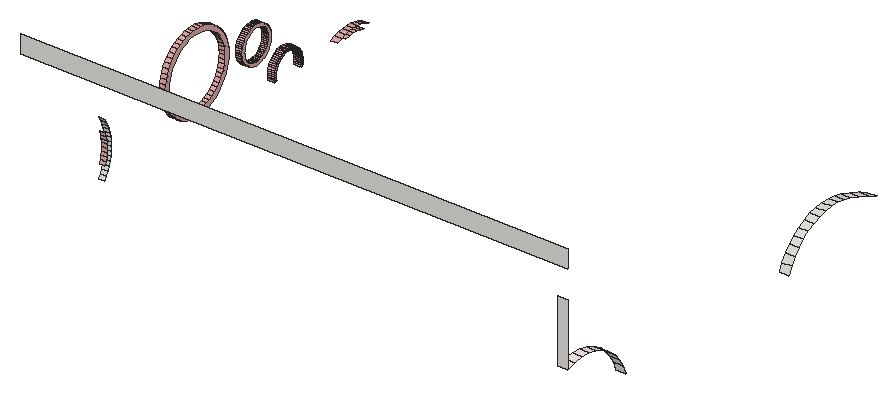
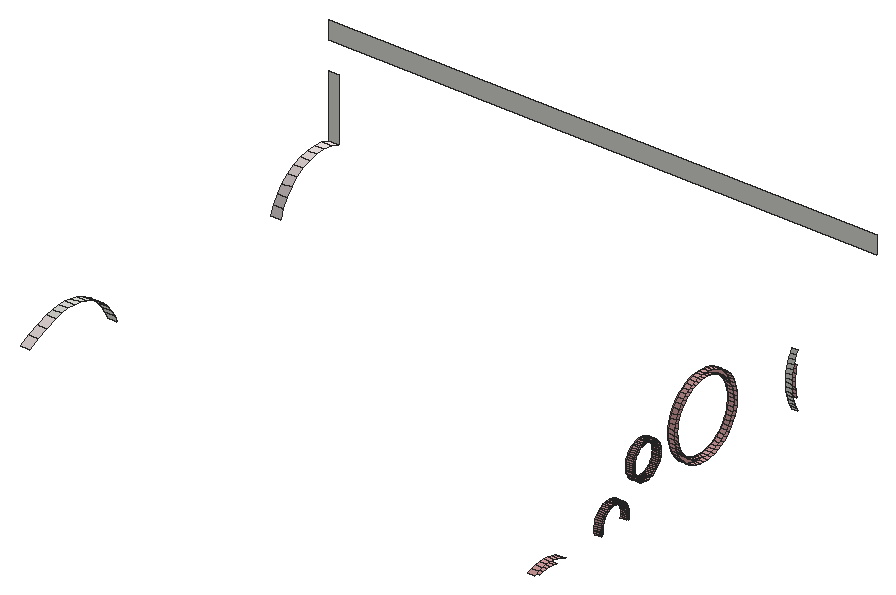
# SketchUp Ruby script. Lengths in inches.
U = 1.inch
M = Sketchup.active_model
def pt(a) = Geom::Point3d.new(a.map { |v| v * U })
def face(e, loops, mat)
  f = e.add_face(loops[0].map { |a| pt(a) })
  loops[1..].each { |l| e.add_face(l.map { |a| pt(a) }).erase! }
  f.material = f.back_material = mat if mat
  f
end
# faces: each face lists its corners as indices into pts; further lists are holes
def faces(e, pts, list, mat = nil) = list.each { |f| face(e, (f[0].is_a?(Array) ? f : [f]).map { |l| l.map { |i| pts[i] } }, mat) }
# xy, xz, yz: faces in a plane at the given z, y or x. An outline is a flat list of corners, or four numbers for a rectangle; further outlines are holes
def ring(l) = l.size == 4 ? [[l[0], l[1]], [l[2], l[1]], [l[2], l[3]], [l[0], l[3]]] : l.each_slice(2).to_a
def flat(e, list, mat, &to3) = list.each { |f| face(e, (f[0].is_a?(Array) ? f : [f]).map { |l| ring(l).map { |u, v| to3.(u, v) } }, mat) }
def xy(e, z, list, mat = nil) = flat(e, list, mat) { |x, y| [x, y, z] }
def xz(e, y, list, mat = nil) = flat(e, list, mat) { |x, z| [x, y, z] }
def yz(e, x, list, mat = nil) = flat(e, list, mat) { |y, z| [x, y, z] }
def lines(e, pts, list) = list.each { |a, b| e.add_line(pt(pts[a]), pt(pts[b])) }
# prism: a flat outline (further loops are holes) pulled along v
def prism(e, loops, v, mat = nil)
  f = face(e, loops, mat); d = Geom::Vector3d.new(v.map { |x| x * U })
  f.pushpull(f.normal.samedirection?(d) ? d.length : -d.length)
end
def box(e, o, s, mat = nil) = prism(e, [[o, [o[0] + s[0], o[1], o[2]], [o[0] + s[0], o[1] + s[1], o[2]], [o[0], o[1] + s[1], o[2]]]], [0, 0, s[2]], mat)
def at(x, y, z, deg = 0) = Geom::Transformation.translation(pt([x, y, z])) * Geom::Transformation.rotation(ORIGIN, Z_AXIS, deg.degrees)
def axes(o, x, y, z) = Geom::Transformation.new([*x, 0, *y, 0, *z, 0, *pt(o).to_a, 1])
def part(name) = M.definitions.add(name)
# library, detail: a bought-in or finely detailed component or shape, given as its bounding box
def library(name, o, s) = part(name).tap { |d| box(d.entities, o, s) }
def detail(e, o, s) = box(e.add_group.entities, o, s)
def put(e, d, t, mat = nil) = e.add_instance(d, t).tap { |i| i.material = mat if mat }
def group(e, t, mat = nil) = e.add_group.tap { |g| g.transformation = t; g.material = mat if mat }.entities
root = M.entities
M.materials.add("Generic").color = [224, 169, 169]
M.materials.add("Generic\#2").color = [246, 234, 234]
xz(root,0,[[180.9375,98.88,184.0625,120],[0,129.25,184.0625,135.25]])
xz(root,88.38,[[10.6875,99.81,12.9375,100.3125]],"Generic")
xz(root,89.3,[[10.6875,99.77,12.9375,100.36]],"Generic")
xz(root,101.73,[[10.6875,86.95,12.9375,87.45]],"Generic")
xz(root,102.58,[[10.6875,86.91,12.9375,87.49]],"Generic")
yz(root,12.625,[[[59.06,89.02,60.53,89.17,61.96,89.47,63.36,89.93,64.7,90.54,65.96,91.29,67.13,92.18,68.2,93.1875,69.15,94.31,69.97,95.53,70.65,96.83,71.18,98.2,71.5625,99.62,71.78,101.07,71.84,102.54,71.74,104,71.48,105.45,71.06,106.86,70.49,108.21,69.77,109.49,68.92,110.6875,67.93,111.78,66.84,112.76,65.64,113.62,64.36,114.33,63.01,114.9,61.6,115.32,60.15,115.58,58.6875,115.68,57.22,115.62,55.77,115.4,54.35,115.02,52.98,114.48,51.68,113.8,50.46,112.98,49.34,112.03,48.33,110.96,47.44,109.79,46.69,108.53,46.08,107.19,45.625,105.8,45.32,104.36,45.18,102.89,45.2,101.43,45.39,99.97,45.73,98.54,46.22,97.16,46.87,95.84,47.66,94.6,48.58,93.45,49.62,92.41,50.76,91.49,52,90.71,53.32,90.0625,54.71,89.57,56.14,89.23,57.6,89.04],[59,90.55,57.7,90.5625,56.41,90.72,55.14,91.03,53.92,91.47,52.75,92.04,51.65,92.73,50.63,93.55,49.71,94.47,48.9,95.48,48.2,96.58,47.63,97.75,47.1875,98.97,46.89,100.24,46.72,101.53,46.71,102.83,46.83,104.13,47.1,105.4,47.5,106.64,48.04,107.82,48.71,108.94,49.49,109.98,50.39,110.93,51.38,111.77,52.46,112.49,53.61,113.1,54.82,113.57,56.08,113.91,57.37,114.11,58.67,114.16,59.96,114.07,61.25,113.84,62.49,113.47,63.69,112.96,64.83,112.33,65.89,111.57,66.86,110.7,67.73,109.74,68.48,108.68,69.12,107.54,69.625,106.34,70,105.1,70.23,103.81,70.32,102.52,70.27,101.22,70.07,99.93,69.73,98.67,69.26,97.46,68.66,96.31,67.93,95.23,67.09,94.23,66.15,93.34,65.11,92.55,63.99,91.89,62.81,91.35,61.57,90.94,60.3,90.67]]],"Generic")
yz(root,12.9375,[[[83.09,93.93,83.68,93.94,84.26,94.02,84.84,94.15,85.4,94.33,85.9375,94.57,86.45,94.86,86.93,95.2,87.38,95.58,87.79,96.01,88.16,96.47,88.48,96.97,88.75,97.49,88.97,98.04,89.14,98.6,89.25,99.18,89.3,99.77,89.3,100.36,89.24,100.95,89.12,101.53,88.95,102.09,88.72,102.64,88.44,103.16,88.12,103.65,87.75,104.11,87.33,104.53,86.88,104.9,86.39,105.24,85.875,105.52,85.33,105.75,84.77,105.93,84.19,106.06,83.61,106.125,83.02,106.13,82.43,106.09,81.85,105.99,81.28,105.83,80.73,105.62,80.2,105.35,79.7,105.04,79.24,104.68,78.81,104.27,78.42,103.83,78.07,103.35,77.78,102.84,77.53,102.3,77.34,101.74,77.2,101.17,77.12,100.59,77.09,100,77.125,99.41,77.21,98.82,77.36,98.25,77.56,97.7,77.81,97.16,78.11,96.66,78.46,96.18,78.85,95.74,79.29,95.34,79.76,94.99,80.26,94.68,80.79,94.42,81.34,94.21,81.91,94.0625,82.5,93.97],[83.1,94.84,82.6,94.88,82.11,94.96,81.625,95.09,81.15,95.26,80.7,95.48,80.28,95.75,79.875,96.05,79.51,96.39,79.17,96.76,78.875,97.16,78.62,97.6,78.41,98.05,78.24,98.52,78.11,99.01,78.04,99.5,78.01,100,78.03,100.5,78.1,101,78.22,101.49,78.38,101.96,78.59,102.42,78.84,102.85,79.14,103.26,79.47,103.63,79.83,103.98,80.23,104.28,80.65,104.55,81.1,104.78,81.57,104.96,82.05,105.09,82.55,105.18,83.04,105.22,83.55,105.21,84.04,105.15,84.53,105.04,85.01,104.89,85.47,104.69,85.91,104.45,86.33,104.17,86.71,103.85,87.0625,103.49,87.38,103.1,87.66,102.6875,87.89,102.24,88.08,101.78,88.23,101.3,88.33,100.81,88.38,100.3125,88.38,99.81,88.34,99.31,88.24,98.82,88.1,98.34,87.92,97.87,87.69,97.43,87.41,97.01,87.1,96.61,86.75,96.25,86.37,95.93,85.96,95.64,85.52,95.39,85.07,95.19,84.59,95.03,84.1,94.92,83.6,94.86]]],"Generic")
p = [[10.6875,102.25,85.2],[10.6875,102.42,85.76],[12.9375,102.42,85.76],[12.9375,102.25,85.2],[10.6875,126.82,85.59],[10.6875,128.27,85.21],
  [12.9375,128.27,85.21],[12.9375,126.82,85.59],[10.6875,90.64,85.98],[10.6875,90.78,85.41],[12.9375,90.78,85.41],[12.9375,90.64,85.98],
  [10.6875,120.85,85.41],[10.6875,122.32,85.72],[12.9375,122.32,85.72],[12.9375,120.85,85.41],[10.6875,101.59,85.95],[10.6875,101.45,85.47],
  [12.9375,101.45,85.47],[12.9375,101.59,85.95],[10.6875,118.89,86.29],[10.6875,117.37,85.6],[12.9375,117.37,85.6],[12.9375,118.89,86.29],
  [10.6875,125.33,85.81],[12.9375,125.33,85.81],[10.6875,91.59,85.66],[10.6875,91.47,86.14],[12.9375,91.47,86.14],[12.9375,91.59,85.66],
  [10.6875,123.82,85.85],[12.9375,123.82,85.85],[10.6875,102.53,86.33],[12.9375,102.53,86.33],[10.6875,90.55,86.55],[12.9375,90.55,86.55],
  [10.6875,101.6875,86.45],[12.9375,101.6875,86.45],[10.6875,130.28,85.99],[10.6875,128.72,86.59],[12.9375,128.72,86.59],[12.9375,130.28,85.99],
  [10.6875,91.39,86.64],[12.9375,91.39,86.64],[184.0625,94.18,88.68],[184.0625,93.05,86.35],[180.9375,93.05,86.35],[180.9375,94.18,88.68],
  [10.6875,102.58,86.91],[12.9375,102.58,86.91],[10.6875,120.48,86.8125],[12.9375,120.48,86.8125],[10.6875,101.73,86.95],[12.9375,101.73,86.95],
  [10.6875,90.52,87.13],[12.9375,90.52,87.13],[10.6875,91.36,87.14],[12.9375,91.36,87.14],[10.6875,127.1,87.01],[12.9375,127.1,87.01],
  [10.6875,122.11,87.15],[12.9375,122.11,87.15],[10.6875,19.58,86.91],[10.6875,20.3,88.11],[12.625,20.3,88.11],[12.625,19.58,86.91],
  [184.0625,24.39,86.97],[184.0625,23.27,89.8],[180.9375,23.27,89.8],[180.9375,24.39,86.97],[10.6875,125.45,87.25],[12.9375,125.45,87.25],
  [10.6875,90.54,87.72],[12.9375,90.54,87.72],[10.6875,91.39,87.64],[12.9375,91.39,87.64],[10.6875,123.78,87.29],[12.9375,123.78,87.29],
  [10.6875,101.68,87.95],[10.6875,101.73,87.45],[12.9375,101.73,87.45],[12.9375,101.68,87.95],[10.6875,102.58,87.49],[10.6875,102.52,88.07],
  [12.9375,102.52,88.07],[12.9375,102.58,87.49],[10.6875,91.45,88.14],[12.9375,91.45,88.14],[10.6875,90.625,88.29],[12.9375,90.625,88.29],
  [10.6875,101.58,88.4375],[12.9375,101.58,88.4375],[10.6875,20.92,89.36],[12.625,20.92,89.36],[10.6875,91.57,88.625],[12.9375,91.57,88.625],
  [10.6875,102.4,88.64],[12.9375,102.4,88.64],[10.6875,90.76,88.86],[12.9375,90.76,88.86],[10.6875,101.43,88.92],[12.9375,101.43,88.92],
  [10.6875,91.74,89.1],[12.9375,91.74,89.1],[10.6875,102.23,89.2],[12.9375,102.23,89.2],[184.0625,95.59,90.85],[180.9375,95.59,90.85],
  [10.6875,90.95,89.41],[12.9375,90.95,89.41],[10.6875,101.24,89.38],[12.9375,101.24,89.38],[10.6875,56.14,89.23],[10.6875,57.6,89.04],
  [12.625,57.6,89.04],[12.625,56.14,89.23],[10.6875,59.06,89.02],[12.625,59.06,89.02],[10.6875,60.53,89.17],[12.625,60.53,89.17],
  [10.6875,91.94,89.55],[12.9375,91.94,89.55],[10.6875,54.71,89.57],[12.625,54.71,89.57],[10.6875,61.96,89.47],[12.625,61.96,89.47],
  [10.6875,102.01,89.74],[12.9375,102.01,89.74],[10.6875,21.44,90.66],[12.625,21.44,90.66],[10.6875,91.19,89.94],[12.9375,91.19,89.94],
  [10.6875,101.01,89.82],[12.9375,101.01,89.82],[10.6875,63.36,89.93],[12.625,63.36,89.93],[10.6875,53.32,90.0625],[12.625,53.32,90.0625],
  [10.6875,92.2,89.99],[12.9375,92.2,89.99],[10.6875,101.73,90.26],[12.9375,101.73,90.26],[184.0625,21.69,92.4],[180.9375,21.69,92.4],
  [10.6875,100.73,90.24],[12.9375,100.73,90.24],[10.6875,64.7,90.54],[12.625,64.7,90.54],[10.6875,91.49,90.45],[12.9375,91.49,90.45],
  [10.6875,92.49,90.39],[12.9375,92.49,90.39],[10.6875,52,90.71],[12.625,52,90.71],[10.6875,100.41,90.63],[12.9375,100.41,90.63],
  [10.6875,101.41,90.74],[12.9375,101.41,90.74],[10.6875,91.83,90.92],[12.9375,91.83,90.92],[10.6875,92.82,90.77],[12.9375,92.82,90.77],
  [10.6875,59,90.55],[10.6875,57.7,90.5625],[12.625,57.7,90.5625],[12.625,59,90.55],[10.6875,60.3,90.67],[12.625,60.3,90.67],
  [10.6875,65.96,91.29],[12.625,65.96,91.29],[10.6875,56.41,90.72],[12.625,56.41,90.72],[10.6875,100.0625,90.99],[12.9375,100.0625,90.99],
  [10.6875,21.84,92],[12.625,21.84,92],[10.6875,50.76,91.49],[12.625,50.76,91.49],[10.6875,55.14,91.03],[12.625,55.14,91.03],
  [10.6875,61.57,90.94],[12.625,61.57,90.94],[10.6875,101.04,91.19],[12.9375,101.04,91.19],[10.6875,93.18,91.11],[12.9375,93.18,91.11],
  [10.6875,62.81,91.35],[12.625,62.81,91.35],[10.6875,92.21,91.36],[12.9375,92.21,91.36],[184.0625,97.26,92.84],[180.9375,97.26,92.84],
  [10.6875,53.92,91.47],[12.625,53.92,91.47],[10.6875,99.68,91.31],[12.9375,99.68,91.31],[10.6875,93.58,91.42],[12.9375,93.58,91.42],
  [10.6875,20.29,92.4],[10.6875,19.92,91.19],[12.625,19.92,91.19],[12.625,20.29,92.4],[10.6875,100.64,91.61],[12.9375,100.64,91.61],
  [10.6875,63.99,91.89],[12.625,63.99,91.89],[10.6875,67.13,92.18],[12.625,67.13,92.18],[10.6875,99.26,91.59],[12.9375,99.26,91.59],
  [10.6875,92.63,91.76],[12.9375,92.63,91.76],[10.6875,94,91.6875],[12.9375,94,91.6875],[10.6875,49.62,92.41],[12.625,49.62,92.41],
  [10.6875,52.75,92.04],[12.625,52.75,92.04],[10.6875,98.82,91.83],[12.9375,98.82,91.83],[10.6875,100.1875,91.98],[12.9375,100.1875,91.98],
  [10.6875,94.45,91.91],[12.9375,94.45,91.91],[10.6875,93.1,92.11],[12.9375,93.1,92.11],[10.6875,98.36,92.03],[12.9375,98.36,92.03],
  [10.6875,65.11,92.55],[12.625,65.11,92.55],[10.6875,94.92,92.09],[12.9375,94.92,92.09],[10.6875,22.14,93.37],[12.625,22.14,93.37],
  [10.6875,51.65,92.73],[12.625,51.65,92.73],[10.6875,97.89,92.18],[12.9375,97.89,92.18],[10.6875,99.71,92.3125],[12.9375,99.71,92.3125],
  [10.6875,93.59,92.42],[12.9375,93.59,92.42],[10.6875,95.4,92.23],[12.9375,95.4,92.23],[10.6875,68.2,93.1875],[12.625,68.2,93.1875],
  [10.6875,95.9,92.3125],[12.9375,95.9,92.3125],[10.6875,97.4,92.29],[12.9375,97.4,92.29],[10.6875,96.4,92.35],[12.9375,96.4,92.35],
  [10.6875,96.9,92.34],[12.9375,96.9,92.34],[10.6875,99.19,92.59],[12.9375,99.19,92.59],[184.0625,19.72,94.71],[180.9375,19.72,94.71],
  [10.6875,20.56,93.64],[12.625,20.56,93.64],[10.6875,48.58,93.45],[12.625,48.58,93.45],[10.6875,94.11,92.6875],[12.9375,94.11,92.6875],
  [10.6875,66.15,93.34],[12.625,66.15,93.34],[10.6875,98.66,92.82],[12.9375,98.66,92.82],[10.6875,50.63,93.55],[12.625,50.63,93.55],
  [10.6875,94.65,92.9],[12.9375,94.65,92.9],[184.0625,99.15,94.61],[180.9375,99.15,94.61],[10.6875,98.1,93],[12.9375,98.1,93],
  [10.6875,95.22,93.05],[12.9375,95.22,93.05],[10.6875,97.53,93.12],[12.9375,97.53,93.12],[10.6875,95.79,93.15],[12.9375,95.79,93.15],
  [10.6875,96.95,93.1875],[12.9375,96.95,93.1875],[10.6875,69.15,94.31],[12.625,69.15,94.31],[10.6875,96.37,93.2],[12.9375,96.37,93.2],
  [10.6875,67.09,94.23],[12.625,67.09,94.23],[10.6875,22.3125,94.76],[12.625,22.3125,94.76],[10.6875,47.66,94.6],[12.625,47.66,94.6],
  [10.6875,49.71,94.47],[12.625,49.71,94.47],[10.6875,20.71,94.89],[12.625,20.71,94.89],[10.6875,82.5,93.97],[10.6875,83.09,93.93],
  [12.9375,83.09,93.93],[12.9375,82.5,93.97],[10.6875,83.68,93.94],[12.9375,83.68,93.94],[10.6875,84.26,94.02],[12.9375,84.26,94.02],
  [10.6875,81.91,94.0625],[12.9375,81.91,94.0625],[10.6875,84.84,94.15],[12.9375,84.84,94.15],[10.6875,81.34,94.21],[12.9375,81.34,94.21],
  [10.6875,85.4,94.33],[12.9375,85.4,94.33],[184.0625,129.85,94.12],[184.0625,126.21,95.79],[180.9375,126.21,95.79],[180.9375,129.85,94.12],
  [10.6875,67.93,95.23],[12.625,67.93,95.23],[10.6875,80.79,94.42],[12.9375,80.79,94.42],[10.6875,69.97,95.53],[12.625,69.97,95.53],
  [10.6875,85.9375,94.57],[12.9375,85.9375,94.57],[10.6875,80.26,94.68],[12.9375,80.26,94.68],[10.6875,48.9,95.48],[12.625,48.9,95.48],
  [10.6875,46.87,95.84],[12.625,46.87,95.84],[10.6875,86.45,94.86],[12.9375,86.45,94.86],[184.0625,101.25,96.13],[180.9375,101.25,96.13],
  [184.0625,17.39,96.67],[180.9375,17.39,96.67],[10.6875,79.76,94.99],[12.9375,79.76,94.99],[10.6875,22.375,96.15],[12.625,22.375,96.15],
  [10.6875,83.1,94.84],[10.6875,82.6,94.88],[12.9375,82.6,94.88],[12.9375,83.1,94.84],[10.6875,83.6,94.86],[12.9375,83.6,94.86],
  [10.6875,20.77,96.16],[12.625,20.77,96.16],[10.6875,82.11,94.96],[12.9375,82.11,94.96],[10.6875,84.1,94.92],[12.9375,84.1,94.92],
  [10.6875,84.59,95.03],[12.9375,84.59,95.03],[10.6875,86.93,95.2],[12.9375,86.93,95.2],[10.6875,79.29,95.34],[12.9375,79.29,95.34],
  [10.6875,81.625,95.09],[12.9375,81.625,95.09],[10.6875,85.07,95.19],[12.9375,85.07,95.19],[10.6875,81.15,95.26],[12.9375,81.15,95.26],
  [10.6875,68.66,96.31],[12.625,68.66,96.31],[10.6875,85.52,95.39],[12.9375,85.52,95.39],[10.6875,87.38,95.58],[12.9375,87.38,95.58],
  [10.6875,78.85,95.74],[12.9375,78.85,95.74],[10.6875,80.7,95.48],[12.9375,80.7,95.48],[10.6875,85.96,95.64],[12.9375,85.96,95.64],
  [10.6875,48.2,96.58],[12.625,48.2,96.58],[10.6875,70.65,96.83],[12.625,70.65,96.83],[10.6875,80.28,95.75],[12.9375,80.28,95.75],
  [10.6875,86.37,95.93],[12.9375,86.37,95.93],[10.6875,87.79,96.01],[12.9375,87.79,96.01],[10.6875,78.46,96.18],[12.9375,78.46,96.18],
  [10.6875,79.875,96.05],[12.9375,79.875,96.05],[10.6875,46.22,97.16],[12.625,46.22,97.16],[184.0625,122.48,97.25],[180.9375,122.48,97.25],
  [10.6875,86.75,96.25],[12.9375,86.75,96.25],[10.6875,79.51,96.39],[12.9375,79.51,96.39],[10.6875,88.16,96.47],[12.9375,88.16,96.47],
  [184.0625,103.52,97.38],[180.9375,103.52,97.38],[10.6875,20.72,97.42],[12.625,20.72,97.42],[10.6875,22.32,97.55],[12.625,22.32,97.55],
  [10.6875,78.11,96.66],[12.9375,78.11,96.66],[10.6875,69.26,97.46],[12.625,69.26,97.46],[10.6875,87.1,96.61],[12.9375,87.1,96.61],
  [10.6875,79.17,96.76],[12.9375,79.17,96.76],[10.6875,88.48,96.97],[12.9375,88.48,96.97],[10.6875,47.63,97.75],[12.625,47.63,97.75],
  [10.6875,87.41,97.01],[12.9375,87.41,97.01],[184.0625,14.78,98.22],[180.9375,14.78,98.22],[10.6875,77.81,97.16],[12.9375,77.81,97.16],
  [10.6875,71.18,98.2],[12.625,71.18,98.2],[10.6875,78.875,97.16],[12.9375,78.875,97.16],[10.6875,87.69,97.43],[12.9375,87.69,97.43],
  [10.6875,88.75,97.49],[12.9375,88.75,97.49],[10.6875,45.73,98.54],[12.625,45.73,98.54],[10.6875,77.56,97.7],[12.9375,77.56,97.7],
  [10.6875,78.62,97.6],[12.9375,78.62,97.6],[184.0625,118.6875,98.51],[180.9375,118.6875,98.51],[10.6875,20.56,98.68],[12.625,20.56,98.68],
  [10.6875,87.92,97.87],[12.9375,87.92,97.87],[184.0625,105.93,98.35],[180.9375,105.93,98.35],[10.6875,69.73,98.67],[12.625,69.73,98.67],
  [10.6875,88.97,98.04],[12.9375,88.97,98.04],[10.6875,22.14,98.94],[12.625,22.14,98.94],[10.6875,78.41,98.05],[12.9375,78.41,98.05],
  [10.6875,47.1875,98.97],[12.625,47.1875,98.97],[10.6875,77.36,98.25],[12.9375,77.36,98.25],[10.6875,88.1,98.34],[12.9375,88.1,98.34],
  [10.6875,78.24,98.52],[12.9375,78.24,98.52],[10.6875,89.14,98.6],[12.9375,89.14,98.6],[184.0625,11.95,99.33],[180.9375,11.95,99.33],
  [10.6875,71.5625,99.62],[12.625,71.5625,99.62],[10.6875,77.21,98.82],[12.9375,77.21,98.82],[10.6875,88.24,98.82],[12.9375,88.24,98.82],
  [184.0625,108.43,99.01],[180.9375,108.43,99.01],[10.6875,45.39,99.97],[12.625,45.39,99.97],[10.6875,78.11,99.01],[12.9375,78.11,99.01],
  [184.0625,116.17,99.11],[180.9375,116.17,99.11],[10.6875,89.25,99.18],[12.9375,89.25,99.18],[10.6875,20.3,99.91],[12.625,20.3,99.91],
  [10.6875,70.07,99.93],[12.625,70.07,99.93],[10.6875,77.125,99.41],[12.9375,77.125,99.41],[10.6875,88.34,99.31],[12.9375,88.34,99.31],
  [184.0625,2.92,99.73],[184.0625,0,98.88],[180.9375,0,98.88],[180.9375,2.92,99.73],[10.6875,21.85,100.31],[12.625,21.85,100.31],
  [10.6875,46.89,100.24],[12.625,46.89,100.24],[10.6875,78.04,99.5],[12.9375,78.04,99.5],[184.0625,111,99.36],[180.9375,111,99.36],
  [184.0625,113.59,99.4],[180.9375,113.59,99.4],[10.6875,89.3,99.77],[12.9375,89.3,99.77],[184.0625,8.97,99.96],[180.9375,8.97,99.96],
  [10.6875,88.38,99.81],[12.9375,88.38,99.81],[10.6875,77.09,100],[12.9375,77.09,100],[10.6875,78.01,100],[12.9375,78.01,100],
  [10.6875,71.78,101.07],[12.625,71.78,101.07],[184.0625,5.9375,100.09],[180.9375,5.9375,100.09],[10.6875,19.94,101.125],[12.625,19.94,101.125],
  [10.6875,70.27,101.22],[12.625,70.27,101.22],[10.6875,45.2,101.43],[12.625,45.2,101.43],[10.6875,77.12,100.59],[12.9375,77.12,100.59],
  [10.6875,78.03,100.5],[12.9375,78.03,100.5],[10.6875,46.72,101.53],[12.625,46.72,101.53],[10.6875,21.45,101.65],[12.625,21.45,101.65],
  [10.6875,88.33,100.81],[10.6875,88.38,100.3125],[12.9375,88.38,100.3125],[12.9375,88.33,100.81],[10.6875,89.3,100.36],[10.6875,89.24,100.95],
  [12.9375,89.24,100.95],[12.9375,89.3,100.36],[10.6875,78.1,101],[12.9375,78.1,101],[10.6875,77.2,101.17],[12.9375,77.2,101.17],
  [10.6875,88.23,101.3],[12.9375,88.23,101.3],[10.6875,89.12,101.53],[12.9375,89.12,101.53],[10.6875,78.22,101.49],[12.9375,78.22,101.49],
  [10.6875,71.84,102.54],[12.625,71.84,102.54],[10.6875,70.32,102.52],[12.625,70.32,102.52],[10.6875,77.34,101.74],[12.9375,77.34,101.74],
  [10.6875,88.08,101.78],[12.9375,88.08,101.78],[10.6875,45.18,102.89],[12.625,45.18,102.89],[10.6875,46.71,102.83],[12.625,46.71,102.83],
  [10.6875,78.38,101.96],[12.9375,78.38,101.96],[10.6875,88.95,102.09],[12.9375,88.95,102.09],[10.6875,20.9375,102.95],[12.625,20.9375,102.95],
  [10.6875,77.53,102.3],[12.9375,77.53,102.3],[10.6875,87.89,102.24],[12.9375,87.89,102.24],[10.6875,78.59,102.42],[12.9375,78.59,102.42],
  [10.6875,88.72,102.64],[12.9375,88.72,102.64],[10.6875,87.66,102.6875],[12.9375,87.66,102.6875],[10.6875,77.78,102.84],[12.9375,77.78,102.84],
  [10.6875,78.84,102.85],[12.9375,78.84,102.85],[10.6875,70.23,103.81],[12.625,70.23,103.81],[10.6875,71.74,104],[12.625,71.74,104],
  [10.6875,88.44,103.16],[12.9375,88.44,103.16],[10.6875,87.38,103.1],[12.9375,87.38,103.1],[10.6875,46.83,104.13],[12.625,46.83,104.13],
  [10.6875,78.07,103.35],[12.9375,78.07,103.35],[10.6875,79.14,103.26],[12.9375,79.14,103.26],[10.6875,45.32,104.36],[12.625,45.32,104.36],
  [10.6875,20.32,104.21],[12.625,20.32,104.21],[10.6875,87.0625,103.49],[12.9375,87.0625,103.49],[10.6875,88.12,103.65],[12.9375,88.12,103.65],
  [10.6875,78.42,103.83],[12.9375,78.42,103.83],[10.6875,79.47,103.63],[12.9375,79.47,103.63],[10.6875,86.71,103.85],[12.9375,86.71,103.85],
  [10.6875,79.83,103.98],[12.9375,79.83,103.98],[10.6875,87.75,104.11],[12.9375,87.75,104.11],[10.6875,70,105.1],[12.625,70,105.1],
  [10.6875,78.81,104.27],[12.9375,78.81,104.27],[10.6875,86.33,104.17],[12.9375,86.33,104.17],[10.6875,71.48,105.45],[12.625,71.48,105.45],
  [10.6875,80.23,104.28],[12.9375,80.23,104.28],[10.6875,47.1,105.4],[12.625,47.1,105.4],[10.6875,87.33,104.53],[12.9375,87.33,104.53],
  [10.6875,19.6,105.4],[12.625,19.6,105.4],[10.6875,85.91,104.45],[12.9375,85.91,104.45],[10.6875,79.24,104.68],[12.9375,79.24,104.68],
  [10.6875,80.65,104.55],[12.9375,80.65,104.55],[10.6875,45.625,105.8],[12.625,45.625,105.8],[10.6875,85.47,104.69],[12.9375,85.47,104.69],
  [10.6875,86.88,104.9],[12.9375,86.88,104.9],[10.6875,81.1,104.78],[12.9375,81.1,104.78],[10.6875,79.7,105.04],[12.9375,79.7,105.04],
  [10.6875,85.01,104.89],[12.9375,85.01,104.89],[10.6875,81.57,104.96],[12.9375,81.57,104.96],[10.6875,84.53,105.04],[12.9375,84.53,105.04],
  [10.6875,86.39,105.24],[12.9375,86.39,105.24],[10.6875,80.2,105.35],[12.9375,80.2,105.35],[10.6875,82.05,105.09],[12.9375,82.05,105.09],
  [10.6875,84.04,105.15],[12.9375,84.04,105.15],[10.6875,69.625,106.34],[12.625,69.625,106.34],[10.6875,82.55,105.18],[12.9375,82.55,105.18],
  [10.6875,83.55,105.21],[12.9375,83.55,105.21],[10.6875,83.04,105.22],[12.9375,83.04,105.22],[10.6875,85.875,105.52],[12.9375,85.875,105.52],
  [10.6875,47.5,106.64],[12.625,47.5,106.64],[10.6875,71.06,106.86],[12.625,71.06,106.86],[10.6875,80.73,105.62],[12.9375,80.73,105.62],
  [10.6875,85.33,105.75],[12.9375,85.33,105.75],[10.6875,81.28,105.83],[12.9375,81.28,105.83],[10.6875,46.08,107.19],[12.625,46.08,107.19],
  [10.6875,81.85,105.99],[12.9375,81.85,105.99],[10.6875,84.77,105.93],[12.9375,84.77,105.93],[10.6875,84.19,106.06],[12.9375,84.19,106.06],
  [10.6875,82.43,106.09],[12.9375,82.43,106.09],[10.6875,83.02,106.13],[12.9375,83.02,106.13],[10.6875,83.61,106.125],[12.9375,83.61,106.125],
  [10.6875,69.12,107.54],[12.625,69.12,107.54],[10.6875,48.04,107.82],[12.625,48.04,107.82],[10.6875,70.49,108.21],[12.625,70.49,108.21],
  [10.6875,46.69,108.53],[12.625,46.69,108.53],[10.6875,68.48,108.68],[12.625,68.48,108.68],[10.6875,48.71,108.94],[12.625,48.71,108.94],
  [10.6875,69.77,109.49],[12.625,69.77,109.49],[10.6875,47.44,109.79],[12.625,47.44,109.79],[10.6875,67.73,109.74],[12.625,67.73,109.74],
  [10.6875,49.49,109.98],[12.625,49.49,109.98],[10.6875,68.92,110.6875],[12.625,68.92,110.6875],[10.6875,66.86,110.7],[12.625,66.86,110.7],
  [10.6875,48.33,110.96],[12.625,48.33,110.96],[10.6875,50.39,110.93],[12.625,50.39,110.93],[10.6875,65.89,111.57],[12.625,65.89,111.57],
  [10.6875,67.93,111.78],[12.625,67.93,111.78],[10.6875,51.38,111.77],[12.625,51.38,111.77],[10.6875,49.34,112.03],[12.625,49.34,112.03],
  [10.6875,64.83,112.33],[12.625,64.83,112.33],[10.6875,52.46,112.49],[12.625,52.46,112.49],[10.6875,66.84,112.76],[12.625,66.84,112.76],
  [10.6875,50.46,112.98],[12.625,50.46,112.98],[10.6875,63.69,112.96],[12.625,63.69,112.96],[10.6875,53.61,113.1],[12.625,53.61,113.1],
  [10.6875,65.64,113.62],[12.625,65.64,113.62],[10.6875,51.68,113.8],[12.625,51.68,113.8],[10.6875,62.49,113.47],[12.625,62.49,113.47],
  [10.6875,54.82,113.57],[12.625,54.82,113.57],[10.6875,61.25,113.84],[12.625,61.25,113.84],[10.6875,56.08,113.91],[12.625,56.08,113.91],
  [10.6875,64.36,114.33],[12.625,64.36,114.33],[10.6875,52.98,114.48],[12.625,52.98,114.48],[10.6875,59.96,114.07],[12.625,59.96,114.07],
  [10.6875,57.37,114.11],[12.625,57.37,114.11],[10.6875,58.67,114.16],[12.625,58.67,114.16],[10.6875,63.01,114.9],[12.625,63.01,114.9],
  [10.6875,54.35,115.02],[12.625,54.35,115.02],[10.6875,61.6,115.32],[12.625,61.6,115.32],[10.6875,55.77,115.4],[12.625,55.77,115.4],
  [10.6875,60.15,115.58],[12.625,60.15,115.58],[10.6875,57.22,115.62],[12.625,57.22,115.62],[10.6875,58.6875,115.68],[12.625,58.6875,115.68]]
faces(root,p,[[0,1,2,3],[4,5,6,7],[8,9,10,11],[12,13,14,15],[16,17,18,19],[20,21,22,23],[24,4,7,25],[26,27,28,29],
  [13,30,31,14],[1,32,33,2],[30,24,25,31],[34,8,11,35],[36,16,19,37],[38,39,40,41],[27,42,43,28],[32,48,49,33],
  [50,20,23,51],[52,36,37,53],[54,34,35,55],[42,56,57,43],[39,58,59,40],[60,50,51,61],[58,70,71,59],[72,54,55,73],
  [56,74,75,57],[76,60,61,77],[70,76,77,71],[78,79,80,81],[82,83,84,85],[74,86,87,75],[88,72,73,89],[90,78,81,91],
  [86,94,95,87],[83,96,97,84],[98,88,89,99],[100,90,91,101],[94,102,103,95],[96,104,105,97],[108,98,99,109],[110,100,101,111],
  [112,113,114,115],[113,116,117,114],[116,118,119,117],[102,120,121,103],[122,112,115,123],[118,124,125,119],[104,126,127,105],[130,108,109,131],
  [132,110,111,133],[124,134,135,125],[136,122,123,137],[120,138,139,121],[126,140,141,127],[144,132,133,145],[134,146,147,135],[148,130,131,149],
  [138,150,151,139],[152,136,137,153],[154,144,145,155],[140,156,157,141],[158,148,149,159],[150,160,161,151],[162,163,164,165],[166,162,165,167],
  [146,168,169,147],[163,170,171,164],[172,154,155,173],[176,152,153,177],[170,178,179,171],[180,166,167,181],[156,182,183,157],[160,184,185,161],
  [186,180,181,187],[188,158,159,189],[178,192,193,179],[194,172,173,195],[184,196,197,185],[198,199,200,201],[182,202,203,183],[204,186,187,205],
  [168,206,207,169],[208,194,195,209],[210,188,189,211],[196,212,213,197],[214,176,177,215],[192,216,217,193],[218,208,209,219],[202,220,221,203],
  [212,222,223,213],[224,210,211,225],[226,218,219,227],[228,204,205,229],[222,230,231,223],[216,234,235,217],[236,226,227,237],[220,238,239,221],
  [240,224,225,241],[230,242,243,231],[206,244,245,207],[242,246,247,243],[248,236,237,249],[246,250,251,247],[250,252,253,251],[252,248,249,253],
  [238,254,255,239],[258,198,201,259],[260,214,215,261],[262,240,241,263],[264,228,229,265],[254,266,267,255],[234,268,269,235],[270,262,263,271],
  [266,274,275,267],[276,270,271,277],[274,278,279,275],[280,276,277,281],[278,282,283,279],[244,284,285,245],[286,280,281,287],[282,286,287,283],
  [288,264,265,289],[292,260,261,293],[268,294,295,269],[296,258,259,297],[298,299,300,301],[299,302,303,300],[302,304,305,303],[306,298,301,307],
  [304,308,309,305],[310,306,307,311],[308,312,313,309],[318,288,289,319],[320,310,311,321],[284,322,323,285],[312,324,325,313],[326,320,321,327],
  [294,328,329,295],[330,292,293,331],[324,332,333,325],[338,326,327,339],[342,343,344,345],[346,342,345,347],[348,296,297,349],[343,350,351,344],
  [352,346,347,353],[354,352,353,355],[332,356,357,333],[358,338,339,359],[350,360,361,351],[362,354,355,363],[360,364,365,361],[366,318,319,367],
  [368,362,363,369],[356,370,371,357],[372,358,359,373],[364,374,375,365],[376,368,369,377],[328,378,379,329],[322,380,381,323],[374,382,383,375],
  [384,376,377,385],[370,386,387,371],[388,372,373,389],[382,390,391,383],[392,330,331,393],[396,384,385,397],[390,398,399,391],[386,400,401,387],
  [404,348,349,405],[408,388,389,409],[410,366,367,411],[412,396,397,413],[398,414,415,399],[400,416,417,401],[378,418,419,379],[420,412,413,421],
  [424,408,409,425],[380,426,427,381],[414,428,429,415],[430,420,421,431],[416,432,433,417],[434,392,393,435],[436,424,425,437],[428,438,439,429],
  [442,404,405,443],[444,430,431,445],[448,410,411,449],[432,450,451,433],[438,454,455,439],[418,456,457,419],[458,436,437,459],[460,444,445,461],
  [454,462,463,455],[450,464,465,451],[426,468,469,427],[470,458,459,471],[472,460,461,473],[476,434,435,477],[462,478,479,463],[464,482,483,465],
  [484,442,443,485],[486,448,449,487],[488,470,471,489],[490,472,473,491],[456,498,499,457],[478,500,501,479],[482,506,507,483],[510,490,491,511],
  [512,488,489,513],[500,514,515,501],[468,516,517,469],[520,484,485,521],[522,486,487,523],[524,476,477,525],[526,512,513,527],[514,528,529,515],
  [498,530,531,499],[534,535,536,537],[538,539,540,541],[528,542,543,529],[544,526,527,545],[546,534,537,547],[539,548,549,540],[542,550,551,543],
  [516,552,553,517],[554,522,523,555],[556,544,545,557],[558,546,547,559],[560,524,525,561],[530,562,563,531],[550,564,565,551],[548,566,567,549],
  [570,556,557,571],[572,558,559,573],[564,574,575,565],[566,576,577,567],[578,572,573,579],[580,570,571,581],[574,582,583,575],[584,554,555,585],
  [552,586,587,553],[576,588,589,577],[590,578,579,591],[562,592,593,563],[594,580,581,595],[582,596,597,583],[598,560,561,599],[602,590,591,603],
  [588,604,605,589],[606,594,595,607],[596,608,609,597],[610,602,603,611],[608,612,613,609],[604,614,615,605],[616,584,585,617],[618,606,607,619],
  [620,610,611,621],[586,622,623,587],[612,624,625,613],[592,626,627,593],[614,628,629,615],[632,620,621,633],[634,618,619,635],[624,636,637,625],
  [638,598,599,639],[640,632,633,641],[628,642,643,629],[636,644,645,637],[646,634,635,647],[648,640,641,649],[644,650,651,645],[652,648,649,653],
  [642,654,655,643],[656,646,647,657],[650,658,659,651],[660,652,653,661],[662,616,617,663],[658,664,665,659],[666,660,661,667],[664,668,669,665],
  [668,666,667,669],[654,670,671,655],[626,672,673,627],[622,674,675,623],[676,656,657,677],[670,678,679,671],[680,676,677,681],[682,638,639,683],
  [684,680,681,685],[678,686,687,679],[686,688,689,687],[690,684,685,691],[692,690,691,693],[694,692,693,695],[688,694,695,689],[696,662,663,697],
  [672,698,699,673],[674,700,701,675],[702,682,683,703],[704,696,697,705],[698,706,707,699],[700,708,709,701],[710,702,703,711],[712,704,705,713],
  [706,714,715,707],[708,716,717,709],[718,712,713,719],[720,710,711,721],[714,722,723,715],[724,718,719,725],[716,726,727,717],[722,728,729,723],
  [730,720,721,731],[732,724,725,733],[728,734,735,729],[726,736,737,727],[738,730,731,739],[740,732,733,741],[734,742,743,735],[736,744,745,737],
  [746,738,739,747],[748,740,741,749],[742,750,751,743],[752,748,749,753],[750,754,755,751],[744,756,757,745],[758,746,747,759],[760,752,753,761],
  [754,762,763,755],[762,764,765,763],[764,760,761,765],[756,766,767,757],[768,758,759,769],[766,770,771,767],[772,768,769,773],[770,774,775,771],
  [776,772,773,777],[778,776,777,779],[774,778,779,775]],"Generic")
faces(root,p,[[44,45,46,47],[62,63,64,65],[63,92,93,64],[106,44,47,107],[92,128,129,93],[128,174,175,129],[190,106,107,191],[174,232,233,175],
  [272,190,191,273],[232,290,291,233],[334,272,273,335],[290,340,341,291],[402,334,335,403],[340,406,407,341],[446,402,403,447],[406,452,453,407],
  [474,446,447,475],[440,480,481,441],[452,496,497,453],[502,474,475,503],[480,504,505,481],[504,502,503,505],[496,532,533,497],[532,568,569,533],
  [568,600,601,569],[600,630,631,601]])
faces(root,p,[[66,67,68,69],[67,142,143,68],[142,256,257,143],[314,315,316,317],[256,336,337,257],[315,394,395,316],[336,422,423,337],[394,440,441,395],
  [422,466,467,423],[492,493,494,495],[466,508,509,467],[518,492,495,519],[508,518,519,509]],"Generic\#2")
